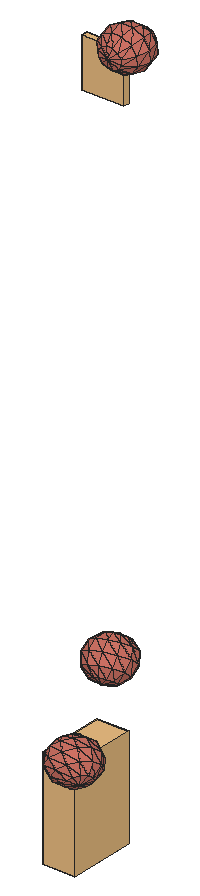
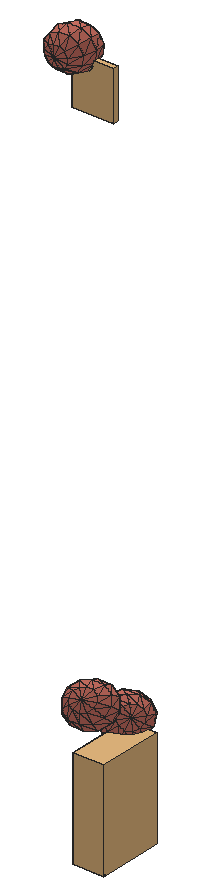
# SketchUp Ruby script. Lengths in inches.
U = 1.inch
M = Sketchup.active_model
def pt(a) = Geom::Point3d.new(a.map { |v| v * U })
def face(e, loops, mat)
  f = e.add_face(loops[0].map { |a| pt(a) })
  loops[1..].each { |l| e.add_face(l.map { |a| pt(a) }).erase! }
  f.material = f.back_material = mat if mat
  f
end
# faces: each face lists its corners as indices into pts; further lists are holes
def faces(e, pts, list, mat = nil) = list.each { |f| face(e, (f[0].is_a?(Array) ? f : [f]).map { |l| l.map { |i| pts[i] } }, mat) }
# xy, xz, yz: faces in a plane at the given z, y or x. An outline is a flat list of corners, or four numbers for a rectangle; further outlines are holes
def ring(l) = l.size == 4 ? [[l[0], l[1]], [l[2], l[1]], [l[2], l[3]], [l[0], l[3]]] : l.each_slice(2).to_a
def flat(e, list, mat, &to3) = list.each { |f| face(e, (f[0].is_a?(Array) ? f : [f]).map { |l| ring(l).map { |u, v| to3.(u, v) } }, mat) }
def xy(e, z, list, mat = nil) = flat(e, list, mat) { |x, y| [x, y, z] }
def xz(e, y, list, mat = nil) = flat(e, list, mat) { |x, z| [x, y, z] }
def yz(e, x, list, mat = nil) = flat(e, list, mat) { |y, z| [x, y, z] }
def lines(e, pts, list) = list.each { |a, b| e.add_line(pt(pts[a]), pt(pts[b])) }
# prism: a flat outline (further loops are holes) pulled along v
def prism(e, loops, v, mat = nil)
  f = face(e, loops, mat); d = Geom::Vector3d.new(v.map { |x| x * U })
  f.pushpull(f.normal.samedirection?(d) ? d.length : -d.length)
end
def box(e, o, s, mat = nil) = prism(e, [[o, [o[0] + s[0], o[1], o[2]], [o[0] + s[0], o[1] + s[1], o[2]], [o[0], o[1] + s[1], o[2]]]], [0, 0, s[2]], mat)
def at(x, y, z, deg = 0) = Geom::Transformation.translation(pt([x, y, z])) * Geom::Transformation.rotation(ORIGIN, Z_AXIS, deg.degrees)
def axes(o, x, y, z) = Geom::Transformation.new([*x, 0, *y, 0, *z, 0, *pt(o).to_a, 1])
def part(name) = M.definitions.add(name)
# library, detail: a bought-in or finely detailed component or shape, given as its bounding box
def library(name, o, s) = part(name).tap { |d| box(d.entities, o, s) }
def detail(e, o, s) = box(e.add_group.entities, o, s)
def put(e, d, t, mat = nil) = e.add_instance(d, t).tap { |i| i.material = mat if mat }
def group(e, t, mat = nil) = e.add_group.tap { |g| g.transformation = t; g.material = mat if mat }.entities
root = M.entities
M.materials.add("green").color = [174, 139, 102]
M.materials.add("vio").color = [206, 114, 100]
c1 = part("3DGeom~239_Defintion")
p = [[90.53,-63.37,-491.99],[67.74,-328.31,-318.83],[-81.52,-183.54,-449.92],[266.4,-189.55,-367.41],[200.76,100.79,-448.8],[-109.61,79.79,-484.74],
  [-45.97,174.5625,-459.8],[-208.9375,10.41,-460.45],[-280.37,201.57,-347.6],[-269.29,-227.52,-333.86],[-317.35,-14.98,-393.44],[-35.07,269.34,-392.33],
  [-149.08,-379.1,-184.82],[393.68,0,-317.54],[219.63,264.9375,-331.92],[-317.35,-14.98,-393.44],[-269.29,-227.52,-333.86],[-422.46,-183.54,-174.92],
  [-317.35,-14.98,-393.44],[-405.78,10.41,-301.68],[-405.78,10.41,-301.68],[-79.84,338.72,-300.39],[-79.84,338.72,-300.39],[219.63,264.9375,-331.92],
  [-35.07,269.34,-392.33],[266.4,-189.55,-367.41],[198.85,-385.11,-102.31],[67.74,-328.31,-318.83],[266.4,-189.55,-367.41],[370.9,-264.9375,-144.38],
  [393.68,0,-317.54],[370.9,-264.9375,-144.38],[266.4,-189.55,-367.41],[-450.55,79.79,-209.74],[-280.37,201.57,-347.6],[-439.65,174.5625,-142.26],
  [-280.37,201.57,-347.6],[-376.01,269.34,-117.33],[-280.37,201.57,-347.6],[-276.68,338.72,-141.62],[-280.37,201.57,-347.6],[-168.27,364.11,-208.62],
  [-276.68,338.72,-141.62],[-168.27,364.11,-208.62],[-280.37,201.57,-347.6],[-269.29,-227.52,-333.86],[-149.08,-379.1,-184.82],[-325.95,-328.31,-1.29],
  [-269.29,-227.52,-333.86],[415.48,189.55,-182.59],[142.09,385.11,-172.68],[415.48,189.55,-182.59],[219.63,264.9375,-331.92],[-79.84,338.72,-300.39],
  [219.63,264.9375,-331.92],[67.74,-328.31,-318.83],[11.08,-429.09,13.74],[-149.08,-379.1,-184.82],[67.74,-328.31,-318.83],[393.68,0,-317.54],
  [481.125,-100.79,-101.2],[370.9,-264.9375,-144.38],[415.48,189.55,-182.59],[393.68,0,-317.54],[-500,-63.37,-15.68],[-168.27,364.11,-208.62],
  [-79.84,338.72,-300.39],[-481.125,100.79,101.2],[-11.08,429.09,-13.74],[-168.27,364.11,-208.62],[-168.27,364.11,-208.62],[-149.08,-379.1,-184.82],
  [-142.09,-385.11,172.68],[-149.08,-379.1,-184.82],[-325.95,-328.31,-1.29],[415.48,189.55,-182.59],[500,63.37,15.68],[325.95,328.31,1.29],
  [415.48,189.55,-182.59],[325.95,328.31,1.29],[415.48,189.55,-182.59],[-415.48,-189.55,182.59],[276.68,-338.72,141.62],[376.01,-269.34,117.33],
  [376.01,-269.34,117.33],[370.9,-264.9375,-144.38],[-370.9,264.9375,144.38],[-370.9,264.9375,144.38],[-376.01,269.34,-117.33],[-198.85,385.11,102.31],
  [-376.01,269.34,-117.33],[-370.9,264.9375,144.38],[168.27,-364.11,208.62],[439.65,-174.5625,142.26],[376.01,-269.34,117.33],[-393.68,0,317.54],
  [149.08,379.1,184.82],[-325.95,-328.31,-1.29],[-219.63,-264.9375,331.93],[-325.95,-328.31,-1.29],[-219.63,-264.9375,331.93],[-415.48,-189.55,182.59],
  [325.95,328.31,1.29],[422.46,183.54,174.92],[149.08,379.1,184.82],[325.95,328.31,1.29],[79.84,-338.72,300.39],[450.55,-79.79,209.74],
  [-266.4,189.55,367.41],[-266.4,189.55,367.41],[-370.9,264.9375,144.38],[-67.74,328.31,318.83],[276.68,-338.72,141.62],[376.01,-269.34,117.33],
  [280.37,-201.57,347.6],[376.01,-269.34,117.33],[280.37,-201.57,347.6],[280.37,-201.57,347.6],[280.37,-201.57,347.6],[-266.4,189.55,367.41],
  [35.07,-269.34,392.33],[-219.63,-264.9375,331.93],[35.07,-269.34,392.33],[405.78,-10.41,301.68],[269.29,227.52,333.86],[149.08,379.1,184.82],
  [-415.48,-189.55,182.59],[-219.63,-264.9375,331.93],[-200.76,-100.78,448.8],[-415.48,-189.55,182.59],[-393.68,0,317.54],[-67.74,328.31,318.83],
  [269.29,227.52,333.86],[149.08,379.1,184.82],[79.84,-338.72,300.39],[168.27,-364.11,208.62],[280.37,-201.57,347.6],[280.37,-201.57,347.6],
  [35.07,-269.34,392.33],[79.84,-338.72,300.39],[280.37,-201.57,347.6],[405.78,-10.41,301.68],[317.35,14.98,393.44],[280.37,-201.57,347.6],
  [317.35,14.98,393.44],[-393.68,0,317.54],[-90.53,63.37,491.99],[-393.68,0,317.54],[-266.4,189.55,367.41],[-266.4,189.55,367.41],
  [81.52,183.54,449.92],[-67.74,328.31,318.83],[-67.74,328.31,318.83],[269.29,227.52,333.86],[45.97,-174.5625,459.8],[317.35,14.98,393.44],
  [269.29,227.52,333.86],[280.37,-201.57,347.6],[109.61,-79.79,484.74],[280.37,-201.57,347.6],[208.9375,-10.41,460.45],[280.37,-201.57,347.6],
  [317.35,14.98,393.44],[280.37,-201.57,347.6],[-266.4,189.55,367.41],[317.35,14.98,393.44]]
faces(c1.entities,p,[[0,1,2],[0,3,1],[4,3,0],[5,0,2],[6,0,5],[6,4,0],[5,2,7],[5,7,8],
  [6,5,8],[7,9,10],[7,2,9],[7,10,8],[11,4,6],[11,6,8],[2,12,9],[2,1,12],
  [4,13,3],[14,13,4],[11,14,4],[15,16,17],[18,17,19],[10,20,8],[21,11,8],[22,23,24],
  [25,26,27],[28,29,26],[30,31,32],[19,33,34],[33,35,36],[35,37,38],[37,39,40],[41,21,8],
  [42,43,44],[45,46,47],[48,47,17],[14,49,13],[50,51,52],[53,50,54],[55,56,57],[58,26,56],
  [59,60,61],[62,60,63],[19,17,64],[19,64,33],[65,50,66],[33,64,67],[33,67,35],[42,68,69],
  [70,68,50],[71,56,72],[73,72,74],[75,76,60],[77,76,78],[50,79,80],[17,47,81],[17,81,64],
  [68,79,50],[29,82,26],[29,83,82],[60,84,85],[35,67,86],[35,87,37],[88,89,42],[42,89,68],
  [90,91,89],[26,92,56],[26,82,92],[60,93,94],[76,93,60],[64,81,95],[64,95,67],[68,96,79],
  [89,96,68],[97,72,98],[99,100,101],[102,103,76],[104,103,105],[56,106,72],[56,92,106],[76,107,93],
  [103,107,76],[67,95,108],[67,109,110],[91,111,89],[89,111,96],[112,113,114],[115,93,116],[92,82,117],
  [93,107,118],[91,119,111],[72,120,121],[72,106,122],[103,123,107],[124,123,103],[125,124,103],[126,127,128],
  [129,128,130],[131,132,133],[134,135,136],[107,123,137],[138,139,140],[141,142,143],[124,144,123],[145,128,146],
  [147,146,148],[149,150,151],[152,150,153],[127,138,154],[127,154,128],[150,155,156],[154,138,157],[158,154,159],
  [160,158,161],[162,160,163],[164,146,150],[150,160,165],[128,154,158],[128,158,146],[146,160,150],[146,158,160]],"vio")
c2 = library("3DGeom~163_Defintion",[-333.59,-500,-156.82],[667.18,1000,313.64])
c3 = part("3DGeom~164_Defintion")
p = [[-316.7,-484.43,-156.82],[-330.53,-495.14,-131.21],[-331.78,-487.36,-147.01],[-300.37,-489.29,-150.82],[-330.53,-495.14,-131.21],[-316.7,-484.43,-156.82],
  [-300.37,-489.29,-150.82],[-316.7,-484.43,-156.82],[-307.47,-486.03,-155.8],[-316.7,-484.43,-156.82],[-331.78,-487.36,-147.01],[-325.6,-484.92,-153.6],
  [-299.12,-497.07,-135.02],[-330.53,-495.14,-131.21],[-300.37,-489.29,-150.82],[-299.12,-497.07,-135.02],[-300.37,-489.29,-150.82],[-297.3125,-493.33,-143.21],
  [-330.53,-495.14,-131.21],[-333.59,-491.1,-138.82],[-331.78,-487.36,-147.01],[-314.2,-500,-125.21],[-330.53,-495.14,-131.21],[-299.12,-497.07,-135.02],
  [-314.2,-500,-125.21],[-299.12,-497.07,-135.02],[-305.3,-499.51,-128.43],[-330.53,-495.14,-131.21],[-314.2,-500,-125.21],[-323.43,-498.4,-126.23],
  [306.85,495.99,152.28],[330.06,486.75,126.11],[323.43,491.02,121.57],[306.85,495.99,152.28],[323.43,491.02,121.57],[315.47,495.38,121.75],
  [306.85,495.99,152.28],[315.47,495.38,121.75],[308.3,498.67,126.61],[306.85,495.99,152.28],[333.59,483.72,134.16],[330.06,486.75,126.11],
  [306.85,495.99,152.28],[308.3,498.67,126.61],[303.86,500,134.83],[306.85,495.99,152.28],[333.05,482.74,143.56],[333.59,483.72,134.16],
  [306.85,495.99,152.28],[303.86,500,134.83],[303.33,499.02,144.23],[306.85,495.99,152.28],[328.61,484.07,151.78],[333.05,482.74,143.56],
  [306.85,495.99,152.28],[321.44,487.36,156.64],[328.61,484.07,151.78],[306.85,495.99,152.28],[313.48,491.72,156.82],[321.44,487.36,156.64]]
faces(c3.entities,p,[[0,1,2],[3,4,5],[6,7,8],[9,10,11],[12,13,14],[15,16,17],[18,19,20],[21,22,23],
  [24,25,26],[27,28,29],[30,31,32],[33,34,35],[36,37,38],[39,40,41],[42,43,44],[45,46,47],
  [48,49,50],[51,52,53],[54,55,56],[57,58,59]],"green")
c4 = part("3DGeom~249_Defintion")
p = [[-255.5,94.92,-415.28],[-6.35,103.625,-485.08],[-12.59,-116.1,-481.02],[239.09,-105.72,-421.38],[244.5,84.5625,-424.9],[1.59,295.58,-359.16],
  [-248.62,261.16,-306.23],[-255.5,94.92,-415.28],[-248.62,261.16,-306.23],[-260.91,-95.36,-411.76],[-15.46,-304.71,-348.07],[236.61,-269.07,-306.25],
  [-255.5,94.92,-415.28],[-260.91,-95.36,-411.76],[426.72,-67.02,-248.84],[429.84,42.84,-250.87],[426.72,-67.02,-248.84],[251.38,250.8,-315.85],
  [429.84,42.84,-250.87],[244.5,84.5625,-424.9],[251.38,250.8,-315.85],[239.09,-105.72,-421.38],[425.28,-161.33,-182.37],[236.61,-269.07,-306.25],
  [239.09,-105.72,-421.38],[426.72,-67.02,-248.84],[-436.1875,60.78,-234.21],[-255.5,94.92,-415.28],[-260.91,-95.36,-411.76],[-432.22,156.76,-171.25],
  [-248.62,261.16,-306.23],[-260.91,-95.36,-411.76],[-263.39,-258.71,-296.63],[-439.31,-49.07,-232.18],[-263.39,-258.71,-296.63],[9.11,408.34,-137.01],
  [251.38,250.8,-315.85],[1.59,295.58,-359.16],[-242.11,358.81,-113.84],[1.59,295.58,-359.16],[-248.62,261.16,-306.23],[-242.11,358.81,-113.84],
  [1.59,295.58,-359.16],[-263.39,-258.71,-296.63],[-15.46,-304.71,-348.07],[-14.18,-411.68,-121.86],[-15.46,-304.71,-348.07],[237.72,-361.7,-110.34],
  [-15.46,-304.71,-348.07],[236.61,-269.07,-306.25],[251.38,250.8,-315.85],[433.81,138.82,-187.91],[429.84,42.84,-250.87],[257.89,348.45,-123.46],
  [251.38,250.8,-315.85],[257.89,348.45,-123.46],[251.38,250.8,-315.85],[236.61,-269.07,-306.25],[425.92,-214.8125,-69.26],[237.72,-361.7,-110.34],
  [236.61,-269.07,-306.25],[-428.46,213.14,-60.17],[-242.11,358.81,-113.84],[-263.39,-258.71,-296.63],[-262.28,-351.34,-100.72],[-440.74,-143.38,-165.7],
  [-262.28,-351.34,-100.72],[429.84,42.84,-250.87],[500,-10.36,-9.62],[429.84,42.84,-250.87],[-500,10.36,9.62],[437.57,195.19,-76.83],
  [257.89,348.45,-123.46],[-440.1,-196.87,-52.6],[14.18,411.68,121.86],[-237.72,361.7,110.34],[-242.11,358.81,-113.84],[-237.72,361.7,110.34],
  [262.28,351.34,100.72],[257.89,348.45,-123.46],[262.28,351.34,100.72],[-262.28,-351.34,-100.72],[-9.11,-408.34,137.01],[242.11,-358.81,113.84],
  [-425.92,214.8125,69.26],[-237.72,361.7,110.34],[237.72,-361.7,-110.34],[428.46,-213.14,60.17],[237.72,-361.7,-110.34],[242.11,-358.81,113.84],
  [-262.28,-351.34,-100.72],[-257.89,-348.45,123.46],[-257.89,-348.45,123.46],[440.1,196.87,52.6],[262.28,351.34,100.72],[-437.57,-195.19,76.83],
  [432.22,-156.76,171.25],[436.1875,-60.78,234.21],[439.31,49.07,232.18],[440.74,143.38,165.7],[-433.81,-138.82,187.91],[-429.84,-42.84,250.87],
  [-426.72,67.02,248.84],[-425.28,161.33,182.37],[263.39,258.71,296.63],[263.39,258.71,296.63],[262.28,351.34,100.72],[242.11,-358.81,113.84],
  [-251.38,-250.8,315.85],[15.46,304.71,348.07],[263.39,258.71,296.63],[-236.61,269.07,306.25],[-236.61,269.07,306.25],[-237.72,361.7,110.34],
  [248.62,-261.16,306.23],[242.11,-358.81,113.84],[248.62,-261.16,306.23],[-236.61,269.07,306.25],[-257.89,-348.45,123.46],[-1.59,-295.58,359.16],
  [-257.89,-348.45,123.46],[-1.59,-295.58,359.16],[-251.38,-250.8,315.85],[248.62,-261.16,306.23],[-1.59,-295.58,359.16],[260.91,95.36,411.76],
  [260.91,95.36,411.76],[263.39,258.71,296.63],[248.62,-261.16,306.23],[-244.5,-84.5625,424.9],[-244.5,-84.5625,424.9],[255.5,-94.92,415.28],
  [255.5,-94.92,415.28],[260.91,95.36,411.76],[248.62,-261.16,306.23],[255.5,-94.92,415.28],[-429.84,-42.84,250.87],[-239.09,105.73,421.38],
  [-426.72,67.02,248.84],[-239.09,105.73,421.38],[-429.84,-42.84,250.87],[-244.5,-84.5625,424.9],[-239.09,105.73,421.38],[12.59,116.1,481.02],
  [260.91,95.36,411.76],[263.39,258.71,296.63],[263.39,258.71,296.63],[15.46,304.71,348.07],[-1.59,-295.58,359.16],[248.62,-261.16,306.23],
  [255.5,-94.92,415.28],[-239.09,105.73,421.38],[15.46,304.71,348.07],[-236.61,269.07,306.25],[-251.38,-250.8,315.85],[6.35,-103.625,485.08],
  [-251.38,-250.8,315.85],[-239.09,105.73,421.38],[15.46,304.71,348.07],[-239.09,105.73,421.38]]
faces(c4.entities,p,[[0,1,2],[1,3,2],[1,4,3],[5,4,1],[6,1,7],[8,5,1],[9,2,10],[2,11,10],
  [2,3,11],[12,2,13],[4,14,3],[4,15,16],[17,18,19],[5,20,4],[21,22,23],[24,25,22],
  [26,27,28],[29,27,26],[29,30,27],[31,10,32],[33,28,34],[26,28,33],[35,36,37],[38,39,40],
  [41,35,42],[43,44,45],[46,47,45],[48,49,47],[50,51,52],[53,51,54],[35,55,56],[57,58,59],
  [60,22,58],[61,30,29],[61,62,30],[63,45,64],[65,34,66],[33,34,65],[25,67,68],[69,51,68],
  [22,25,68],[26,33,70],[29,26,70],[33,65,70],[51,71,68],[72,71,51],[58,22,68],[61,29,70],
  [65,66,73],[65,73,70],[74,55,35],[75,35,76],[77,74,35],[78,71,79],[74,80,55],[81,45,82],
  [45,47,83],[45,83,82],[84,62,61],[84,85,62],[86,58,87],[88,87,89],[90,82,91],[73,66,92],
  [71,93,68],[94,93,71],[87,58,68],[84,61,70],[73,92,95],[73,95,70],[96,87,68],[97,96,68],
  [98,97,68],[99,98,68],[93,99,68],[95,100,70],[100,101,70],[101,102,70],[103,84,70],[102,103,70],
  [104,99,93],[105,93,106],[107,87,96],[103,85,84],[95,92,108],[95,108,100],[109,110,80],[109,80,74],
  [103,111,85],[112,74,113],[82,83,114],[115,96,116],[117,109,74],[118,82,119],[120,121,122],[82,123,124],
  [125,98,99],[126,99,127],[128,96,97],[102,111,103],[100,108,129],[100,130,101],[131,97,98],[132,98,133],
  [134,97,135],[136,137,138],[102,139,111],[140,141,142],[143,144,145],[143,146,147],[148,149,150],[151,152,153],
  [154,148,155],[156,155,141],[157,143,158],[148,150,155],[155,150,144],[155,144,143],[141,143,159],[141,155,143]],"vio")
c5 = library("3DGeom~183_Defintion",[-58.28,-500,-420.6],[116.56,1000,841.2])
c6 = part("3DGeom~184_Defintion")
p = [[-21.41,-458.84,-420.6],[-21.53,-500,-365.15],[-53.32,-468.47,-406.125],[10.44,-469.79,-407.35],[-21.53,-500,-365.15],[10.44,-469.79,-407.35],
  [-3.01,-461.98,-417.24],[-53.32,-468.47,-406.125],[-39.83,-461.21,-416.53],[10.38,-490.37,-379.625],[-21.53,-500,-365.15],[10.44,-469.79,-407.35],
  [10.38,-490.37,-379.625],[10.44,-469.79,-407.35],[15.34,-480.18,-393.58],[-53.32,-468.47,-406.125],[-21.53,-500,-365.15],[-53.38,-489.05,-378.4],
  [-53.32,-468.47,-406.125],[-53.38,-489.05,-378.4],[-58.28,-478.66,-392.17],[-21.53,-500,-365.15],[10.38,-490.37,-379.625],[-3.11,-497.625,-369.22],
  [-21.53,-500,-365.15],[-39.93,-496.86,-368.51],[-53.38,-489.05,-378.4],[21.98,487.39,420.6],[20.96,500,348.46],[2.62,499.54,353.65],
  [21.98,487.39,420.6],[39.43,498.77,352.9375],[20.96,500,348.46],[21.98,487.39,420.6],[53.09,496.1875,365.88],[39.43,498.77,352.9375],
  [21.98,487.39,420.6],[2.62,499.54,353.65],[-10.67,497.51,367.11],[21.98,487.39,420.6],[58.28,492.93,383.82],[53.09,496.1875,365.88],
  [21.98,487.39,420.6],[-10.67,497.51,367.11],[-15.34,494.46,385.24],[21.98,487.39,420.6],[53.61,489.88,401.95],[58.28,492.93,383.82],
  [21.98,487.39,420.6],[-15.34,494.46,385.24],[-10.15,491.2,403.18],[21.98,487.39,420.6],[40.32,487.85,415.41],[53.61,489.88,401.95],
  [21.98,487.39,420.6],[-10.15,491.2,403.18],[3.51,488.61,416.12]]
faces(c6.entities,p,[[0,1,2],[3,4,0],[5,0,6],[0,7,8],[9,10,11],[12,13,14],[15,16,17],[18,19,20],
  [21,22,23],[24,25,26],[27,28,29],[30,31,32],[33,34,35],[36,37,38],[39,40,41],[42,43,44],
  [45,46,47],[48,49,50],[51,52,53],[54,55,56]],"green")
c7 = part("3DGeom~215_Defintion")
p = [[153.1,0,-493.4375],[146.71,-288.7,-360.18],[-37.25,-159.0625,-480.02],[311.55,-150.94,-371.8],[-46.38,150.94,-482.85],[302.41,159.0625,-374.64],
  [82.93,288.7,-379.97],[-211.22,13.19,-471.24],[-233.43,261.44,-342.89],[-158.77,340.98,-283.49],[-233.43,261.44,-342.89],[-158.77,340.98,-283.49],
  [-9.49,-389.54,-237.18],[-217.61,-275.51,-337.98],[-9.49,-389.54,-237.18],[-217.61,-275.51,-337.98],[-217.61,-275.51,-337.98],[-367.42,-87.65,-348.23],
  [-328.6,181.91,-336.18],[-367.42,-87.65,-348.23],[-233.43,261.44,-342.89],[-328.6,181.91,-336.18],[142.07,389.54,-190.15],[-124.625,399.2,-173.9],
  [82.93,288.7,-379.97],[-158.77,340.98,-283.49],[142.07,389.54,-190.15],[82.93,288.7,-379.97],[440.86,-13.19,-268.92],[370.7,275.51,-155.45],
  [440.86,-13.19,-268.92],[302.41,159.0625,-374.64],[142.07,389.54,-190.15],[370.7,275.51,-155.45],[311.55,-150.94,-371.8],[291.35,-340.98,-143.84],
  [146.71,-288.7,-360.18],[311.55,-150.94,-371.8],[386.52,-261.44,-150.55],[291.35,-340.98,-143.84],[440.86,-13.19,-268.92],[311.55,-150.94,-371.8],
  [146.71,-288.7,-360.18],[201.17,-399.2,-72.82],[-9.49,-389.54,-237.18],[146.71,-288.7,-360.18],[291.35,-340.98,-143.84],[-367.42,-87.65,-348.23],
  [-339.66,-318.125,-105.38],[-473.12,-124.56,-146.79],[-217.61,-275.51,-337.98],[-418.78,123.69,-265.17],[-328.6,181.91,-336.18],[-367.42,-87.65,-348.23],
  [-418.78,123.69,-265.17],[-233.43,261.44,-342.89],[-328.6,181.91,-336.18],[-357.93,301.89,-111.05],[-233.43,261.44,-342.89],[-357.93,301.89,-111.05],
  [-217.61,-275.51,-337.98],[-115.19,-426.45,-35.74],[-339.66,-318.125,-105.38],[-217.61,-275.51,-337.98],[-357.93,301.89,-111.05],[440.86,-13.19,-268.92],
  [461.18,-181.91,-91.15],[500,87.65,-79.1],[440.86,-13.19,-268.92],[370.7,275.51,-155.45],[440.86,-13.19,-268.92],[-479.8,102.38,-148.87],
  [140.14,-420.51,43.48],[115.19,426.45,35.74],[370.7,275.51,-155.45],[-140.14,420.51,-43.48],[-357.93,301.89,-111.05],[339.66,318.125,105.38],
  [370.7,275.51,-155.45],[339.66,318.125,105.38],[370.7,275.51,-155.45],[291.35,-340.98,-143.84],[357.93,-301.89,111.05],[357.93,-301.89,111.05],
  [-500,-87.65,79.1],[-495.32,123.69,-18.45],[-370.7,-275.51,155.45],[357.93,-301.89,111.05],[-461.18,181.91,91.15],[-386.52,261.44,150.55],
  [-291.35,340.98,143.84],[-201.17,399.2,72.82],[-357.93,301.89,-111.05],[-291.35,340.98,143.84],[-357.93,301.89,-111.05],[-339.66,-318.125,-105.38],
  [-142.07,-389.54,190.15],[-339.66,-318.125,-105.38],[-142.07,-389.54,190.15],[-370.7,-275.51,155.45],[495.32,-123.69,18.45],[357.93,-301.89,111.05],
  [473.12,124.56,146.79],[339.66,318.125,105.38],[124.625,-399.2,173.9],[-142.07,-389.54,190.15],[-440.86,13.19,268.92],[479.8,-102.38,148.86],
  [357.93,-301.89,111.05],[9.49,389.54,237.18],[-302.41,-159.0625,374.64],[-302.41,-159.0625,374.64],[-311.55,150.94,371.8],[217.61,275.51,337.98],
  [339.66,318.125,105.38],[217.61,275.51,337.98],[158.77,-340.98,283.49],[233.43,-261.44,342.89],[158.77,-340.98,283.49],[328.6,-181.91,336.18],
  [233.43,-261.44,342.89],[357.93,-301.89,111.05],[418.78,-123.69,265.16],[328.6,-181.91,336.18],[357.93,-301.89,111.05],[357.93,-301.89,111.05],
  [-146.71,288.7,360.18],[-291.35,340.98,143.84],[-146.71,288.7,360.18],[367.42,87.65,348.23],[217.61,275.51,337.98],[-146.71,288.7,360.18],
  [-370.7,-275.51,155.45],[-142.07,-389.54,190.15],[-82.93,-288.7,379.97],[-370.7,-275.51,155.45],[-302.41,-159.0625,374.64],[-142.07,-389.54,190.15],
  [158.77,-340.98,283.49],[-142.07,-389.54,190.15],[158.77,-340.98,283.49],[-82.93,-288.7,379.97],[-146.71,288.7,360.18],[217.61,275.51,337.98],
  [9.49,389.54,237.18],[211.22,-13.19,471.24],[328.6,-181.91,336.18],[418.78,-123.69,265.16],[418.78,-123.69,265.16],[367.42,87.65,348.23],
  [-440.86,13.19,268.92],[-153.09,0,493.4375],[-440.86,13.19,268.92],[-311.55,150.94,371.8],[158.77,-340.98,283.49],[233.43,-261.44,342.89],
  [46.38,-150.94,482.85],[37.25,159.0625,480.02],[367.42,87.65,348.23],[217.61,275.51,337.98],[-146.71,288.7,360.18],[217.61,275.51,337.98],
  [367.42,87.65,348.23],[-311.55,150.94,371.8],[-146.71,288.7,360.18],[-311.55,150.94,371.8]]
faces(c7.entities,p,[[0,1,2],[0,3,1],[4,0,2],[5,3,0],[6,0,4],[6,5,0],[4,2,7],[8,4,7],
  [9,4,10],[11,6,4],[2,12,13],[2,1,14],[7,2,15],[7,16,17],[18,7,19],[20,7,21],
  [22,5,6],[23,24,25],[23,26,27],[5,28,3],[29,30,31],[32,33,5],[34,35,36],[37,38,39],
  [40,38,41],[42,43,44],[45,46,43],[47,48,49],[47,50,48],[51,47,49],[52,53,54],[55,56,57],
  [25,58,59],[60,61,62],[63,44,61],[56,51,57],[23,25,64],[65,66,38],[67,66,68],[69,67,70],
  [51,49,71],[51,71,57],[44,72,61],[44,43,72],[73,74,26],[75,73,26],[75,26,23],[75,23,76],
  [77,67,78],[73,79,80],[81,38,82],[38,66,83],[71,49,84],[71,84,85],[71,85,57],[49,48,86],
  [49,86,84],[43,46,87],[85,88,57],[88,89,57],[89,90,57],[91,75,92],[93,91,94],[95,61,96],
  [97,98,99],[66,100,101],[67,100,66],[102,100,67],[103,102,67],[72,43,87],[91,73,75],[61,104,105],
  [61,72,104],[85,84,106],[85,106,88],[100,107,108],[102,107,100],[109,79,73],[91,109,73],[104,72,87],
  [93,109,91],[84,86,110],[84,111,106],[88,106,112],[88,112,89],[113,102,114],[109,115,79],[116,104,87],
  [117,118,87],[119,120,121],[122,123,124],[107,122,125],[89,126,127],[93,128,109],[129,107,102],[130,129,102],
  [129,122,107],[89,112,131],[132,133,134],[135,134,136],[137,104,138],[139,140,141],[142,143,144],[145,146,147],
  [145,148,149],[150,136,151],[152,151,153],[134,154,155],[156,155,146],[156,146,145],[157,158,159],[160,157,161],
  [134,155,156],[157,145,162],[163,157,164],[165,151,157],[136,134,156],[136,156,151],[151,156,145],[151,145,157]],"vio")
g1 = group(root,at(15.3125,134.49,26.21))
put(g1,c1,axes([-1.05,-1.04,10.17],[0,0.00039,0],[0,0,-0.00039],[-0.00039,0,0]),"vio")
g2 = group(root,at(15.3125,134.49,26.21))
put(g2,c2,axes([-1.18,-0.76,9.74],[0,0.00081,0],[0,0,-0.00081],[-0.00081,0,0]),"green")
put(g2,c3,axes([-1.18,-0.76,9.74],[0,0.00081,0],[0,0,-0.00081],[-0.00081,0,0]),"green")
g3 = group(root,at(15.3125,134.49,26.21))
put(g3,c4,axes([-0.95,-0.63,15.18],[0,0.00039,0],[0,0,-0.00039],[-0.00039,0,0]),"vio")
g4 = group(root,at(15.3125,134.49,26.21))
put(g4,c5,axes([-1.13,-0.625,14.96],[0,0.0004,0],[0,0,-0.0004],[-0.0004,0,0]),"green")
put(g4,c6,axes([-1.13,-0.625,14.96],[0,0.0004,0],[0,0,-0.0004],[-0.0004,0,0]),"green")
g5 = group(root,at(15.3125,134.49,26.21))
put(g5,c7,axes([-1.24,-0.44,10.58],[0,0.00038,0],[0,0,-0.00038],[-0.00038,0,0]),"vio")
